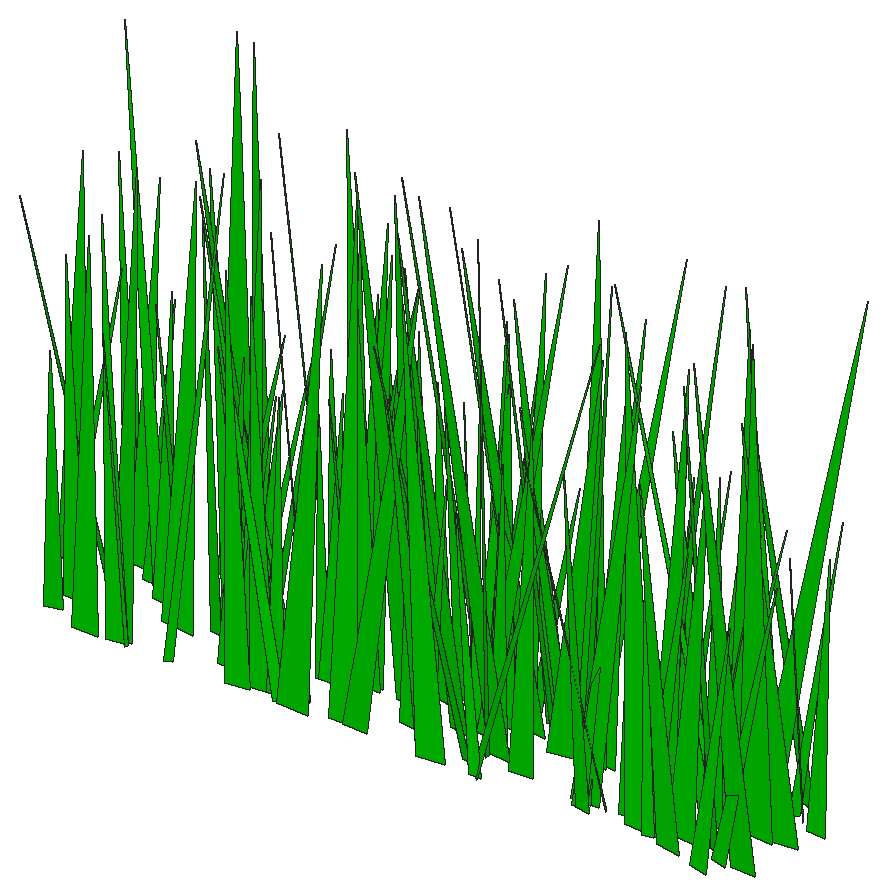
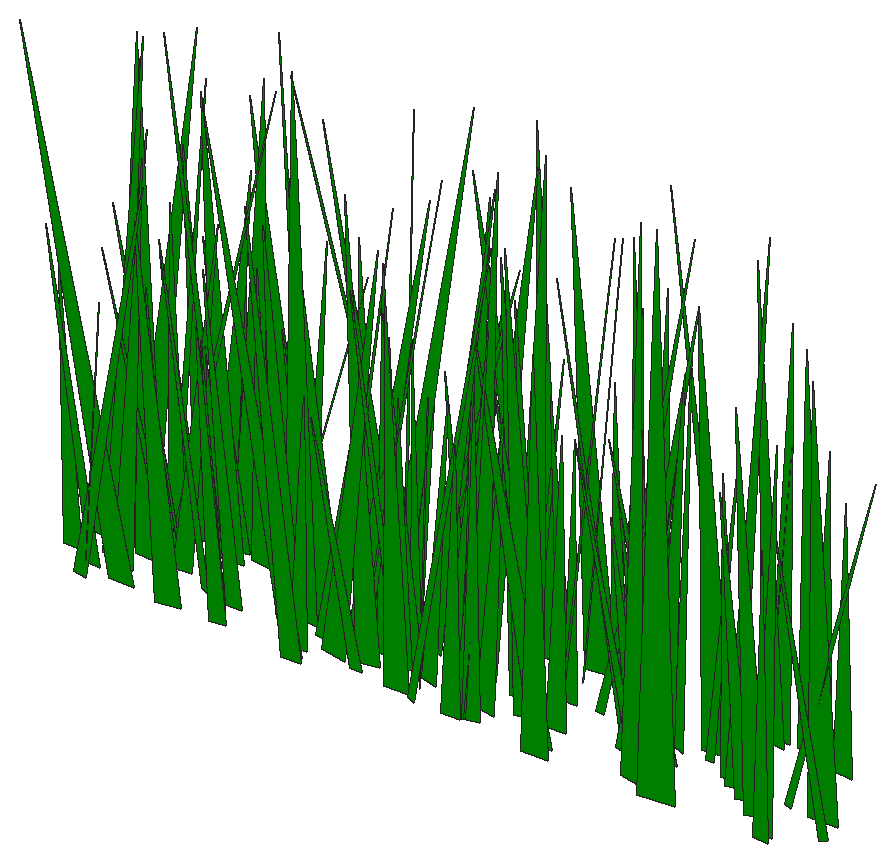
# SketchUp Ruby script. Lengths in inches.
U = 1.inch
M = Sketchup.active_model
def pt(a) = Geom::Point3d.new(a.map { |v| v * U })
def face(e, loops, mat)
  f = e.add_face(loops[0].map { |a| pt(a) })
  loops[1..].each { |l| e.add_face(l.map { |a| pt(a) }).erase! }
  f.material = f.back_material = mat if mat
  f
end
# faces: each face lists its corners as indices into pts; further lists are holes
def faces(e, pts, list, mat = nil) = list.each { |f| face(e, (f[0].is_a?(Array) ? f : [f]).map { |l| l.map { |i| pts[i] } }, mat) }
# xy, xz, yz: faces in a plane at the given z, y or x. An outline is a flat list of corners, or four numbers for a rectangle; further outlines are holes
def ring(l) = l.size == 4 ? [[l[0], l[1]], [l[2], l[1]], [l[2], l[3]], [l[0], l[3]]] : l.each_slice(2).to_a
def flat(e, list, mat, &to3) = list.each { |f| face(e, (f[0].is_a?(Array) ? f : [f]).map { |l| ring(l).map { |u, v| to3.(u, v) } }, mat) }
def xy(e, z, list, mat = nil) = flat(e, list, mat) { |x, y| [x, y, z] }
def xz(e, y, list, mat = nil) = flat(e, list, mat) { |x, z| [x, y, z] }
def yz(e, x, list, mat = nil) = flat(e, list, mat) { |y, z| [x, y, z] }
def lines(e, pts, list) = list.each { |a, b| e.add_line(pt(pts[a]), pt(pts[b])) }
# prism: a flat outline (further loops are holes) pulled along v
def prism(e, loops, v, mat = nil)
  f = face(e, loops, mat); d = Geom::Vector3d.new(v.map { |x| x * U })
  f.pushpull(f.normal.samedirection?(d) ? d.length : -d.length)
end
def box(e, o, s, mat = nil) = prism(e, [[o, [o[0] + s[0], o[1], o[2]], [o[0] + s[0], o[1] + s[1], o[2]], [o[0], o[1] + s[1], o[2]]]], [0, 0, s[2]], mat)
def at(x, y, z, deg = 0) = Geom::Transformation.translation(pt([x, y, z])) * Geom::Transformation.rotation(ORIGIN, Z_AXIS, deg.degrees)
def axes(o, x, y, z) = Geom::Transformation.new([*x, 0, *y, 0, *z, 0, *pt(o).to_a, 1])
def part(name) = M.definitions.add(name)
# library, detail: a bought-in or finely detailed component or shape, given as its bounding box
def library(name, o, s) = part(name).tap { |d| box(d.entities, o, s) }
def detail(e, o, s) = box(e.add_group.entities, o, s)
def put(e, d, t, mat = nil) = e.add_instance(d, t).tap { |i| i.material = mat if mat }
def group(e, t, mat = nil) = e.add_group.tap { |g| g.transformation = t; g.material = mat if mat }.entities
root = M.entities
M.materials.add("[Color G06]").color = [0, 204, 0]
c1 = part("fur_instance\#9")
p = [[0.8125,0,1.79],[0.67,-0.02,1.48],[0,-0.11,0],[0,0.11,0]]
faces(c1.entities,p,[[0,1,2,3]])
put(root,c1,axes([93.84,18.74,4.28],[-3.89646,-0.18346,0.14964],[-1.31582,0.54351,0.0144],[0.09794,0.00319,6.14655]),"[Color G06]")
put(root,c1,axes([91.91,19.62,4.28],[3.12062,-0.14706,0.72615],[-1.08428,-0.43858,0.20488],[-0.41552,0.03998,4.91888]),"[Color G06]")
put(root,c1,axes([92.53,18.83,4.28],[1.07387,-0.64965,0.80947],[-4.689,-0.15045,0.02454],[-0.10555,0.07411,7.14548]),"[Color G06]")
put(root,c1,axes([93.39,20.43,4.28],[-3.09128,0.34495,2.27214],[2.68125,0.45797,0.16142],[1.11426,-0.145,5.91515]),"[Color G06]")
put(root,c1,axes([93.26,20.6875,4.28],[2.09361,-0.28235,1.59317],[-2.08135,-0.31869,-0.37848],[-0.95081,0.07592,4.33654]),"[Color G06]")
put(root,c1,axes([93.93,17.18,4.28],[-1.75667,0.44508,1.20041],[3.248,0.25495,-0.24203],[0.53216,-0.08687,5.43976]),"[Color G06]")
put(root,c1,axes([93.77,16.44,4.28],[0.82028,-0.41002,0.27869],[-2.93084,-0.11631,-0.38855],[-0.3008,0.0152,4.54577]),"[Color G06]")
put(root,c1,axes([94.18,19.75,4.28],[2.44539,-0.44611,2.29894],[-3.47731,-0.3534,0.38435],[-0.71351,0.19338,6.00598]),"[Color G06]")
put(root,c1,axes([95.69,18.84,4.28],[-5.50408,0.262,2.74443],[1.96973,0.80489,-0.00292],[1.73847,-0.08245,8.69235]),"[Color G06]")
put(root,c1,axes([95.28,15.95,4.28],[1.34941,-0.50708,2.74932],[-4.03826,-0.20268,0.13312],[-0.5474,0.24521,5.79546]),"[Color G06]")
put(root,c1,axes([95,19.24,4.28],[1.79163,-0.35089,1.36215],[-2.6566,-0.2517,0.3568],[-0.32427,0.12335,4.60295]),"[Color G06]")
put(root,c1,axes([95.96,18.57,4.28],[-0.05374,0.48445,0.5777],[3.49502,0.00841,-0.08393],[0.06248,-0.05376,5.19231]),"[Color G06]")
put(root,c1,axes([96.32,16.05,4.28],[-3.04819,0.41639,2.40329],[3.21453,0.45082,0.13451],[1.08113,-0.16646,6.37601]),"[Color G06]")
put(root,c1,axes([96.6875,16.03,4.28],[-3.15579,0.00932,1.42542],[0.06585,0.45972,-0.01948],[0.9538,-0.00092,4.71758]),"[Color G06]")
put(root,c1,axes([96.33,16.26,4.28],[-3.10388,-0.45728,3.67036],[-3.73413,0.49252,-0.0047],[1.68554,0.24905,6.74844]),"[Color G06]")
put(root,c1,axes([97.1,18.1,4.28],[-2.89601,-0.2272,1.17344],[-1.61995,0.41776,0.36111],[0.8042,0.02337,4.95312]),"[Color G06]")
put(root,c1,axes([97.35,19.93,4.28],[2.65943,-0.37764,3.84419],[-3.30311,-0.44333,0.10139],[-1.7434,0.26387,5.67195]),"[Color G06]")
put(root,c1,axes([96.87,20.75,4.28],[-0.46085,-0.83837,1.99902],[-6.14945,0.07313,0.35656],[0.3458,0.18322,9.00496]),"[Color G06]")
put(root,c1,axes([97.17,17.6875,4.28],[-0.17926,0.69352,1.04407],[5.01514,0.0299,-0.35804],[0.26688,-0.09602,7.42934]),"[Color G06]")
put(root,c1,axes([98.09,20.3,4.28],[4.00217,0.51365,3.84718],[4.02511,-0.62347,0.20904],[-1.99817,-0.22712,8.12668]),"[Color G06]")
put(root,c1,axes([98.17,18.14,4.28],[-3.68963,-0.24991,2.40579],[-1.95372,0.55064,-0.12218],[1.40925,0.10907,6.12933]),"[Color G06]")
put(root,c1,axes([99.25,19.2,4.28],[-4.23286,-0.41552,1.14239],[-3.02985,0.59449,-0.23743],[0.53229,0.07964,7.73302]),"[Color G06]")
put(root,c1,axes([99.39,18.26,4.28],[-2.77863,0.18738,0.85951],[1.36625,0.39418,-0.00554],[0.51936,-0.03444,4.61299]),"[Color G06]")
put(root,c1,axes([97.85,18.88,4.28],[2.58253,0.33507,0.20383],[2.40581,-0.36019,-0.06949],[-0.06814,-0.0177,5.27169]),"[Color G06]")
put(root,c1,axes([98.71,19.3125,4.28],[0.4572,0.37676,0.22484],[2.70004,-0.0621,-0.31087],[0.18037,-0.02547,4.08373]),"[Color G06]")
put(root,c1,axes([98.13,16.07,4.28],[5.3709,-0.09992,2.06039],[-0.78155,-0.77164,0.25212],[-1.34279,0.04947,8.0944]),"[Color G06]")
put(root,c1,axes([98.83,18.76,4.28],[2.42071,-0.14971,0.92501],[-1.11544,-0.34574,0.09241],[-0.53987,0.04307,3.95671]),"[Color G06]")
put(root,c1,axes([98.25,19.93,4.28],[3.31354,-0.14565,0.46224],[-1.05379,-0.46358,0.09389],[-0.27596,0.02135,5.1917]),"[Color G06]")
put(root,c1,axes([99.64,16.82,4.28],[1.01835,0.43821,1.3594],[3.26496,-0.14454,-0.11097],[-0.20706,-0.12394,4.93596]),"[Color G06]")
put(root,c1,axes([99.76,17.72,4.28],[-3.72194,0.39483,3.39525],[3.10993,0.58083,-0.14391],[1.87244,-0.17988,6.98793]),"[Color G06]")
put(root,c1,axes([101.17,17.85,4.28],[-2.49958,0.14717,0.27971],[1.06861,0.3473,0.34042],[0.083,-0.03945,4.04083]),"[Color G06]")
put(root,c1,axes([100.51,16.16,4.28],[2.10886,-0.45616,3.20377],[-3.71989,-0.33881,-0.07218],[-1.20772,0.24705,5.81658]),"[Color G06]")
put(root,c1,axes([101.93,16.22,4.28],[-5.06722,0.19594,1.09993],[1.42792,0.71307,0.10205],[0.69071,-0.03668,7.85845]),"[Color G06]")
put(root,c1,axes([101.59,19.1,4.28],[-5.31084,-0.10589,2.01226],[-0.80014,0.76313,-0.10405],[1.32255,0.03648,8.01749]),"[Color G06]")
put(root,c1,axes([100.5,16.4,4.28],[-0.03822,0.3921,0.39168],[2.81477,0.00825,-0.33482],[0.22852,-0.036,4.18954]),"[Color G06]")
put(root,c1,axes([101.21,16.4,4.28],[-1.24891,0.53433,1.85989],[4.01862,0.17814,0.14882],[0.28644,-0.16944,6.0216]),"[Color G06]")
put(root,c1,axes([99.85,18.47,4.28],[4.49386,0.1881,1.29104],[1.40867,-0.63487,-0.32669],[-0.76255,-0.06428,7.00486]),"[Color G06]")
put(root,c1,axes([101.05,20.87,4.28],[1.2221,-0.55456,1.65828],[-4.10523,-0.18041,-0.1728],[-0.44017,0.14294,6.21566]),"[Color G06]")
put(root,c1,axes([101.48,19.39,4.28],[-1.12076,0.40498,1.3731],[3.0284,0.16284,0.00434],[0.32794,-0.11967,4.65261]),"[Color G06]")
put(root,c1,axes([101.65,16.42,4.28],[-1.66124,0.33643,2.06365],[2.65178,0.25908,-0.08377],[0.83395,-0.15365,4.3772]),"[Color G06]")
put(root,c1,axes([102.63,16.73,4.28],[-4.7485,-0.04764,2.0607],[-0.40645,0.68838,-0.26382],[1.3611,0.03935,7.11043]),"[Color G06]")
put(root,c1,axes([102.11,17.97,4.28],[-1.88073,0.25132,1.71302],[1.99341,0.28301,0.11917],[0.76688,-0.1193,3.89132]),"[Color G06]")
put(root,c1,axes([101.15,20.4375,4.28],[3.16659,-0.42839,0.35632],[-3.08134,-0.44015,0.37842],[0.00573,0.04849,6.58309]),"[Color G06]")
put(root,c1,axes([102.3,17.92,4.28],[1.97491,-0.32217,1.54539],[-2.46488,-0.28637,0.17834],[-0.57554,0.12094,4.53912]),"[Color G06]")
put(root,c1,axes([103.28,18.34,4.28],[-3.64295,0.61374,2.55132],[4.55965,0.53533,-0.25051],[1.22274,-0.16774,8.53537]),"[Color G06]")
put(root,c1,axes([102.48,19.33,4.28],[2.22897,-0.58177,2.14936],[-4.38582,-0.31691,0.30601],[-0.4883,0.19077,7.06288]),"[Color G06]")
put(root,c1,axes([102.25,19.07,4.28],[1.99857,0.40492,0.53348],[2.92384,-0.27856,-0.17891],[-0.10314,-0.05049,5.26549]),"[Color G06]")
put(root,c1,axes([102.52,16.11,4.28],[1.88857,-0.65611,1.42145],[-4.79811,-0.26231,0.33133],[-0.14461,0.13468,7.57025]),"[Color G06]")
put(root,c1,axes([102.89,18.62,4.28],[3.15118,-0.34018,2.2047],[-2.64489,-0.46328,0.23279],[-1.06388,0.14414,5.9515]),"[Color G06]")
put(root,c1,axes([103.65,19.79,4.28],[0.94362,0.37236,2.29687],[2.98238,-0.16663,0.36634],[-0.77306,-0.18834,4.21692]),"[Color G06]")
put(root,c1,axes([103.63,20.43,4.28],[-2.31668,0.32663,1.96439],[2.50437,0.35016,-0.09102],[0.97071,-0.12386,4.92301]),"[Color G06]")
put(root,c1,axes([104.02,20.43,4.28],[3.20506,0.22319,3.43048],[2.00772,-0.52241,-0.28564],[-1.94915,-0.17111,5.34665]),"[Color G06]")
put(root,c1,axes([103.26,18.58,4.28],[1.08815,0.61742,1.92393],[4.6095,-0.15041,-0.27866],[-0.11883,-0.18062,6.80873]),"[Color G06]")
put(root,c1,axes([104.39,16.76,4.28],[-3.05555,-0.1694,1.31165],[-1.2742,0.43995,-0.1033],[0.78891,0.05447,4.91334]),"[Color G06]")
put(root,c1,axes([104.23,20.58,4.28],[-0.72935,0.42847,0.39469],[3.08165,0.10272,-0.08977],[0.11962,-0.03388,4.71904]),"[Color G06]")
put(root,c1,axes([104.92,18.31,4.28],[-3.50034,-0.63116,1.44018],[-4.58207,0.49629,0.10894],[0.64791,0.09998,8.55095]),"[Color G06]")
put(root,c1,axes([104.16,19.74,4.28],[0.6065,0.40059,1.2176],[2.96966,-0.09305,0.21254],[-0.31248,-0.10677,4.38306]),"[Color G06]")
put(root,c1,axes([105.65,20.55,4.28],[-5.08392,-0.19994,1.23093],[-1.45589,0.7173,-0.04718],[0.78399,0.03546,7.89458]),"[Color G06]")
put(root,c1,axes([104.08,16.37,4.28],[3.78024,-0.5139,3.25161],[-4.03161,-0.56342,0.2407],[-1.43551,0.22907,7.8867]),"[Color G06]")
put(root,c1,axes([105,18.37,4.28],[-3.90686,-0.47181,2.71475],[-3.55337,0.58117,0.18007],[1.4563,0.15231,7.72232]),"[Color G06]")
put(root,c1,axes([105.41,19.07,4.28],[-1.1513,-0.34801,0.18385],[-2.48608,0.16144,0.32846],[0.25112,0.00268,4.09462]),"[Color G06]")
put(root,c1,axes([104.5625,16.3,4.28],[3.26322,0.58149,0.62672],[4.17424,-0.45757,0.22115],[-0.37522,-0.03328,7.91079]),"[Color G06]")
put(root,c1,axes([105.86,19.47,4.28],[-1.80493,-0.31982,1.5233],[-2.46419,0.25903,-0.27472],[0.47607,0.12826,4.35331]),"[Color G06]")
put(root,c1,axes([105.72,18.01,4.28],[-0.99996,-0.40833,1.46825],[-3.06896,0.14759,0.04646],[0.34832,0.12816,4.62441]),"[Color G06]")
put(root,c1,axes([105.63,17.37,4.28],[-0.05933,-0.4049,1.23086],[-3.01624,0.01209,0.13195],[0.10856,0.1145,4.33863]),"[Color G06]")
put(root,c1,axes([105.86,19.89,4.28],[-2.89794,-0.04474,1.74415],[-0.26826,0.4355,0.28776],[1.18019,-0.01087,4.34813]),"[Color G06]")
put(root,c1,axes([106.89,18.01,4.28],[-4.32646,-0.39958,1.55166],[-2.93223,0.61428,-0.09103],[0.83121,0.08716,7.75532]),"[Color G06]")
put(root,c1,axes([106.9,16.56,4.28],[-1.73603,-0.48483,0.62303],[-3.49799,0.24312,-0.03867],[0.16294,0.05363,5.80807]),"[Color G06]")
put(root,c1,axes([108.08,16.84,4.28],[-4.14354,-0.22371,0.26192],[-1.61046,0.57754,-0.24328],[0.10449,0.03,6.63635]),"[Color G06]")
put(root,c1,axes([106.32,20.36,4.28],[1.68964,-0.51335,1.50627],[-3.78885,-0.24416,-0.06559],[-0.46147,0.12509,6.05358]),"[Color G06]")
put(root,c1,axes([107.3,16.23,4.28],[-2.33687,0.59443,1.12124],[4.3128,0.32984,-0.00897],[0.36596,-0.09133,7.26558]),"[Color G06]")
put(root,c1,axes([106.49,17.09,4.28],[1.69106,0.32708,0.82542],[2.36926,-0.24285,0.21197],[-0.43972,-0.05062,4.31653]),"[Color G06]")
put(root,c1,axes([106.93,18.69,4.28],[2.84952,-0.18117,2.01208],[-1.43455,-0.43114,0.07851],[-1.20105,0.08513,4.67996]),"[Color G06]")
put(root,c1,axes([106.9,19.29,4.28],[-0.55988,-0.376,1.22303],[-2.78443,0.09168,0.39041],[0.43244,0.1035,4.09732]),"[Color G06]")
put(root,c1,axes([108.47,19.14,4.28],[-5.45633,0.00868,1.38093],[0.07617,0.77159,0.11494],[0.92292,-0.01235,8.1546]),"[Color G06]")
put(root,c1,axes([106.57,19.22,4.28],[2.97411,-0.29039,1.38472],[-2.17337,-0.4253,0.1816],[-0.6866,0.08839,5.42329]),"[Color G06]")
put(root,c1,axes([108.7,17.54,4.28],[-4.54438,-0.5425,1.27889],[-3.9395,0.63888,-0.13715],[0.58966,0.08741,8.93977]),"[Color G06]")
put(root,c1,axes([106.53,19.92,4.28],[3.64973,0.22583,1.27978],[1.69235,-0.51754,-0.28979],[-0.70134,-0.07365,5.96064]),"[Color G06]")
put(root,c1,axes([108.59,19.24,4.28],[-3.61575,-0.53988,0.70519],[-3.88292,0.50672,0.09206],[0.36722,0.0422,7.91688]),"[Color G06]")
put(root,c1,axes([107.61,19.01,4.28],[0.00779,0.56762,1.84071],[4.25231,0.00159,-0.09651],[0.06511,-0.17174,6.08301]),"[Color G06]")
put(root,c1,axes([108.87,19.9375,4.28],[-2.37359,-0.53051,1.44935],[-3.91541,0.3315,-0.38452],[0.28914,0.13397,6.69085]),"[Color G06]")
put(root,c1,axes([107.8,19.74,4.28],[3.39326,-0.4544,2.29282],[-3.44467,-0.49527,0.11199],[-1.05177,0.15608,7.03039]),"[Color G06]")
put(root,c1,axes([108.41,17.36,4.28],[-5.12554,-0.01683,3.20812],[-0.15515,0.77472,-0.08683],[2.1443,0.01583,7.66213]),"[Color G06]")
put(root,c1,axes([108.83,16.29,4.28],[-2.20919,0.23108,0.8109],[1.65343,0.31639,-0.29527],[0.55373,-0.02282,4.11689]),"[Color G06]")
put(root,c1,axes([109.41,19.09,4.28],[-4.64181,-0.17121,1.58282],[-1.24258,0.66331,0.10232],[1.04166,0.02831,7.17538]),"[Color G06]")
put(root,c1,axes([108.52,17.72,4.28],[-0.83078,-0.35819,2.3901],[-2.99661,0.12946,-0.098],[0.41946,0.21539,4.03372]),"[Color G06]")
put(root,c1,axes([107.87,20.18,4.28],[1.78047,0.29163,0.21438],[2.09625,-0.24784,-0.15951],[-0.01154,-0.02488,4.10192]),"[Color G06]")
put(root,c1,axes([109.64,19.37,4.28],[-2.42513,-0.37739,0.62512],[-2.72515,0.34026,-0.01815],[0.27002,0.04457,5.43119]),"[Color G06]")
put(root,c1,axes([107.6,18.27,4.28],[4.7219,0.41956,0.96343],[3.01362,-0.66382,0.21615],[-0.62168,-0.03117,8.36539]),"[Color G06]")
put(root,c1,axes([109.86,20.23,4.28],[-0.43164,-0.36198,1.06187],[-2.68732,0.06344,0.04426],[0.14679,0.09702,3.93271]),"[Color G06]")
put(root,c1,axes([109.74,17.18,4.28],[1.39004,-0.51169,1.00004],[-3.71949,-0.19761,-0.06648],[-0.27921,0.08502,5.8642]),"[Color G06]")
put(root,c1,axes([109.62,20.85,4.28],[3.72719,-0.40371,1.11323],[-2.9121,-0.52784,-0.21031],[-0.67537,0.048,7.05049]),"[Color G06]")
put(root,c1,axes([109.93,18.7,4.28],[2.82691,-0.56288,0.25439],[-4.03338,-0.39487,-0.24893],[-0.23409,0.0061,7.36108]),"[Color G06]")
put(root,c1,axes([110.85,18.88,4.28],[2.06528,0.7239,2.81119],[5.45783,-0.31005,0.21516],[-0.83621,-0.2358,8.34742]),"[Color G06]")
put(root,c1,axes([108.8,16.33,4.28],[5.50071,0.1682,0.16117],[1.20955,-0.76653,-0.3161],[-0.05995,-0.03203,8.41062]),"[Color G06]")
put(root,c1,axes([109.68,20.7,4.28],[5.20167,-0.33776,0.84086],[-2.43531,-0.72872,0.02608],[-0.50262,0.03533,8.57576]),"[Color G06]")
put(root,c1,axes([112.87,17.05,4.28],[-3.73876,-0.06528,0.13829],[-0.46779,0.52151,0.02745],[0.09409,-0.00094,5.63141]),"[Color G06]")
put(root,c1,axes([111.14,19.05,4.28],[0.48196,0.58411,1.18235],[4.25981,-0.06178,-0.37266],[0.16176,-0.11344,6.29079]),"[Color G06]")
put(root,c1,axes([112.35,16.65,4.28],[2.30153,0.2882,2.78528],[2.42235,-0.37348,-0.03182],[-1.36994,-0.1762,4.62307]),"[Color G06]")
put(root,c1,axes([112.19,17.03,4.28],[2.22369,0.23146,1.45551],[1.76153,-0.32837,-0.01282],[-0.77497,-0.08225,4.14725]),"[Color G06]")
put(root,c1,axes([112.17,16.72,4.28],[1.46127,0.32768,0.12335],[2.34445,-0.20408,0.24019],[-0.18004,0.00208,4.12879]),"[Color G06]")
put(root,c1,axes([112.15,16.92,4.28],[5.21096,0.21408,2.78428],[1.6054,-0.76887,0.07945],[-1.80279,-0.06589,8.11873]),"[Color G06]")
put(root,c1,axes([112.48,20.51,4.28],[1.12034,0.38497,1.44431],[2.92226,-0.15353,-0.36251],[-0.1259,-0.13782,4.43813]),"[Color G06]")
put(root,c1,axes([112.66,19.54,4.28],[-1.75291,-0.33465,2.9458],[-2.78682,0.30878,0.32534],[1.37036,0.19987,4.42977]),"[Color G06]")
put(root,c1,axes([112.83,19.92,4.28],[2.55484,-0.12738,1.18496],[-0.94877,-0.3713,-0.01575],[-0.75024,0.03578,4.0551]),"[Color G06]")
put(root,c1,axes([112.16,17.02,4.28],[3.04677,-0.58146,0.48407],[-4.18116,-0.42481,0.16575],[-0.10131,0.0456,7.71668]),"[Color G06]")
put(root,c1,axes([113.57,17.1875,4.28],[0.83181,0.43858,0.90203],[3.18021,-0.12338,0.34032],[-0.37783,-0.07291,4.85042]),"[Color G06]")
put(root,c1,axes([114.33,16.78,4.28],[-2.04493,0.70183,1.00036],[5.05793,0.29037,-0.30687],[0.44342,-0.07555,8.11361]),"[Color G06]")
put(root,c1,axes([115.81,18.38,4.28],[-5.68424,0.04625,0.82232],[0.35837,0.79527,0.39477],[0.53322,-0.04141,8.50081]),"[Color G06]")
put(root,c1,axes([115.05,18.83,4.28],[-2.85507,0.37784,1.15218],[2.7671,0.40484,0.06547],[0.52841,-0.07851,5.88248]),"[Color G06]")
put(root,c1,axes([113.3,18.86,4.28],[5.39029,0.25763,1.90486],[1.92831,-0.76816,-0.25393],[-1.14868,-0.08057,8.51249]),"[Color G06]")
put(root,c1,axes([113.85,19.31,4.28],[3.30186,0.22,0.98629],[1.585,-0.46882,0.16015],[-0.64212,-0.02596,5.46692]),"[Color G06]")
put(root,c1,axes([114.69,16.64,4.28],[-2.09811,0.20447,1.62788],[1.59843,0.31748,0.02094],[0.88404,-0.08874,3.82564]),"[Color G06]")
put(root,c1,axes([114.39,17.57,4.28],[1.92249,0.61722,2.02641],[4.61326,-0.27245,-0.24328],[-0.38476,-0.18271,7.20833]),"[Color G06]")
put(root,c1,axes([114.16,20.59,4.28],[1.39741,-0.55872,0.02589],[-4.00168,-0.19449,0.3282],[0.20165,0.01236,6.3336]),"[Color G06]")
put(root,c1,axes([114.45,17.02,4.28],[1.97224,-0.37012,0.62773],[-2.68643,-0.27334,0.3395],[-0.06612,0.06594,4.9305]),"[Color G06]")
put(root,c1,axes([115.58,16.41,4.28],[-1.67859,-0.52071,0.65178],[-3.74267,0.23775,0.28889],[0.3559,0.04429,6.11213]),"[Color G06]")
put(root,c1,axes([115.71,18.2,4.28],[1.50614,0.45805,1.73021],[3.43411,-0.22462,0.15358],[-0.5804,-0.14041,5.39864]),"[Color G06]")
put(root,c1,axes([115.72,18.88,4.28],[0.98913,0.3949,0.76092],[2.86887,-0.14111,0.08207],[-0.22043,-0.06445,4.48252]),"[Color G06]")
put(root,c1,axes([115.48,17.13,4.28],[1.29414,-0.56332,0.78329],[-4.07294,-0.17759,0.36011],[0.07157,0.07981,6.32967]),"[Color G06]")
put(root,c1,axes([117.13,20.71,4.28],[-3.83371,-0.32398,0.98479],[-2.33692,0.54116,0.13009],[0.609,0.03712,6.69857]),"[Color G06]")
put(root,c1,axes([116.67,17.1,4.28],[-4.43866,-0.23015,2.23737],[-1.68094,0.65128,0.24703],[1.4627,0.05005,7.07336]),"[Color G06]")
put(root,c1,axes([114.87,19.47,4.28],[3.44829,-0.11803,0.0617],[-0.84141,-0.47972,-0.38333],[-0.10114,-0.03337,5.29286]),"[Color G06]")
put(root,c1,axes([116.49,19.625,4.28],[-2.67291,-0.45752,2.01276],[-3.43096,0.39313,0.08794],[0.89838,0.14014,6.32435]),"[Color G06]")
put(root,c1,axes([115.26,18.59,4.28],[3.38156,-0.00893,0.69191],[-0.04525,-0.47557,-0.21134],[-0.46516,-0.01868,5.05047]),"[Color G06]")
put(root,c1,axes([116.15,18.85,4.28],[-2.07667,-0.58584,3.89106],[-4.81459,0.32879,-0.05301],[1.11724,0.32795,7.00408]),"[Color G06]")
put(root,c1,axes([117.2,19.19,4.28],[-4.85566,0.36657,2.41062],[2.6725,0.70947,-0.36862],[1.53931,-0.07546,8.24414]),"[Color G06]")
put(root,c1,axes([117.03,18.45,4.28],[0.08297,-0.76411,1.51579],[-5.57206,-0.0092,0.14862],[0.08576,0.1416,8.18934]),"[Color G06]")
put(root,c1,axes([117.98,16.75,4.28],[-3.384,-0.56859,1.81074],[-4.20514,0.47969,-0.25117],[0.64069,0.14529,7.91546]),"[Color G06]")
put(root,c1,axes([117.51,19.99,4.28],[-2.62866,-0.04453,1.41071],[-0.28034,0.38938,0.24506],[0.95619,-0.00825,3.95002]),"[Color G06]")
put(root,c1,axes([117.98,18.61,4.28],[-1.62927,-0.59461,1.09174],[-4.3262,0.22439,-0.38241],[0.01825,0.1079,6.81168]),"[Color G06]")
put(root,c1,axes([116.96,16.02,4.28],[0.72661,0.38693,0.32672],[2.77624,-0.09849,-0.39234],[0.19954,-0.03867,4.26899]),"[Color G06]")
put(root,c1,axes([115.9375,20.39,4.28],[4.25918,0.60589,0.59577],[4.36166,-0.59333,-0.33544],[-0.11823,-0.06162,9.08738]),"[Color G06]")
put(root,c1,axes([117.13,20.09,4.28],[3.29566,-0.19754,0.57365],[-1.39541,-0.46251,-0.38827],[-0.45488,-0.01239,5.34729]),"[Color G06]")
put(root,c1,axes([117.16,16.6875,4.28],[2.45927,0.31937,0.41919],[2.30699,-0.34142,-0.35075],[-0.04425,-0.05062,5.01037]),"[Color G06]")
put(root,c1,axes([118.26,19.63,4.28],[0.93195,0.3925,1.04982],[2.89299,-0.1334,-0.00709],[-0.21616,-0.0932,4.43142]),"[Color G06]")
